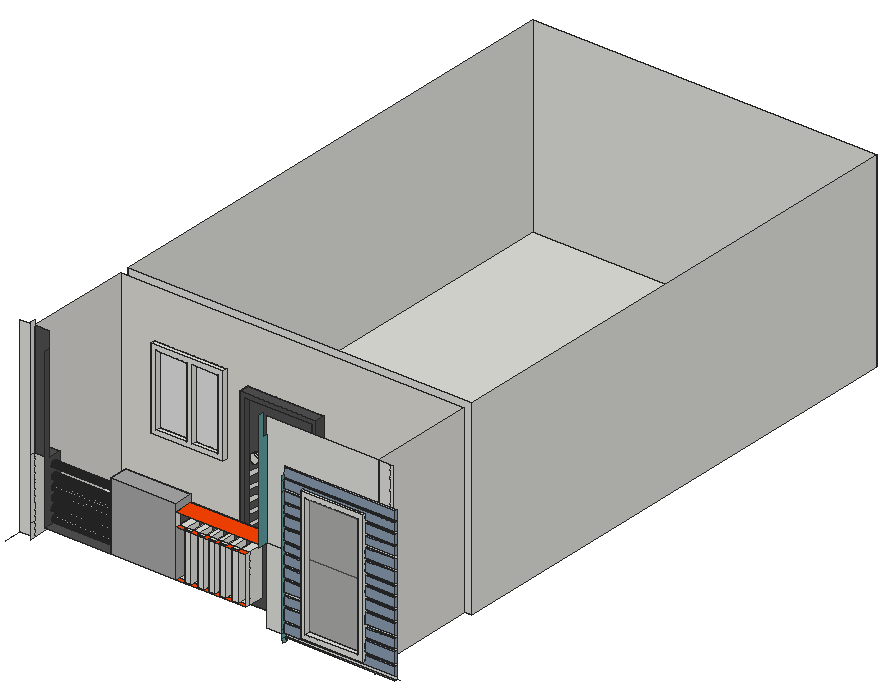
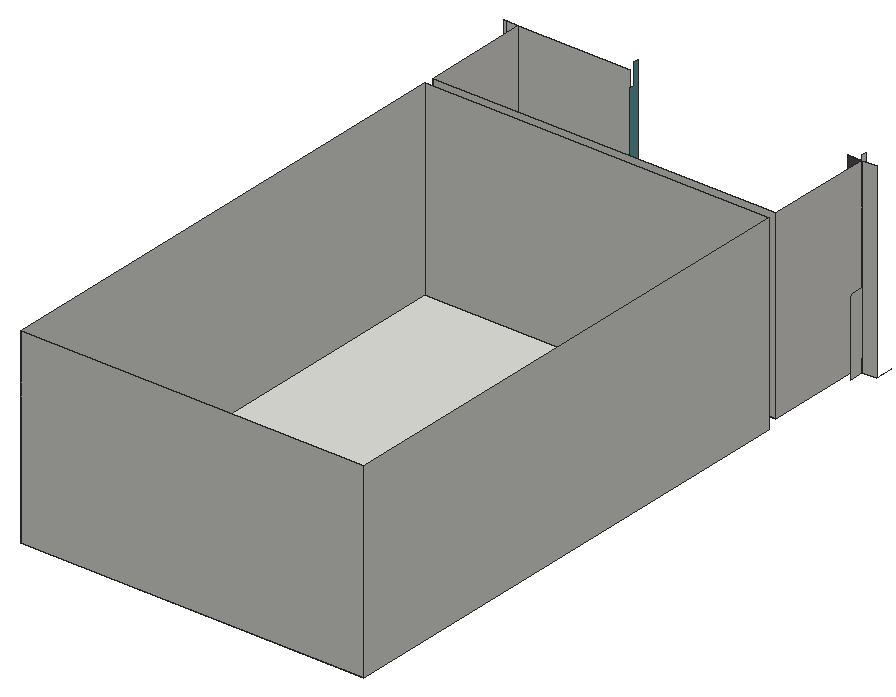
# SketchUp Ruby script. Lengths in inches.
U = 1.inch
M = Sketchup.active_model
def pt(a) = Geom::Point3d.new(a.map { |v| v * U })
def face(e, loops, mat)
  f = e.add_face(loops[0].map { |a| pt(a) })
  loops[1..].each { |l| e.add_face(l.map { |a| pt(a) }).erase! }
  f.material = f.back_material = mat if mat
  f
end
# faces: each face lists its corners as indices into pts; further lists are holes
def faces(e, pts, list, mat = nil) = list.each { |f| face(e, (f[0].is_a?(Array) ? f : [f]).map { |l| l.map { |i| pts[i] } }, mat) }
# xy, xz, yz: faces in a plane at the given z, y or x. An outline is a flat list of corners, or four numbers for a rectangle; further outlines are holes
def ring(l) = l.size == 4 ? [[l[0], l[1]], [l[2], l[1]], [l[2], l[3]], [l[0], l[3]]] : l.each_slice(2).to_a
def flat(e, list, mat, &to3) = list.each { |f| face(e, (f[0].is_a?(Array) ? f : [f]).map { |l| ring(l).map { |u, v| to3.(u, v) } }, mat) }
def xy(e, z, list, mat = nil) = flat(e, list, mat) { |x, y| [x, y, z] }
def xz(e, y, list, mat = nil) = flat(e, list, mat) { |x, z| [x, y, z] }
def yz(e, x, list, mat = nil) = flat(e, list, mat) { |y, z| [x, y, z] }
def lines(e, pts, list) = list.each { |a, b| e.add_line(pt(pts[a]), pt(pts[b])) }
# prism: a flat outline (further loops are holes) pulled along v
def prism(e, loops, v, mat = nil)
  f = face(e, loops, mat); d = Geom::Vector3d.new(v.map { |x| x * U })
  f.pushpull(f.normal.samedirection?(d) ? d.length : -d.length)
end
def box(e, o, s, mat = nil) = prism(e, [[o, [o[0] + s[0], o[1], o[2]], [o[0] + s[0], o[1] + s[1], o[2]], [o[0], o[1] + s[1], o[2]]]], [0, 0, s[2]], mat)
def at(x, y, z, deg = 0) = Geom::Transformation.translation(pt([x, y, z])) * Geom::Transformation.rotation(ORIGIN, Z_AXIS, deg.degrees)
def axes(o, x, y, z) = Geom::Transformation.new([*x, 0, *y, 0, *z, 0, *pt(o).to_a, 1])
def part(name) = M.definitions.add(name)
# library, detail: a bought-in or finely detailed component or shape, given as its bounding box
def library(name, o, s) = part(name).tap { |d| box(d.entities, o, s) }
def detail(e, o, s) = box(e.add_group.entities, o, s)
def put(e, d, t, mat = nil) = e.add_instance(d, t).tap { |i| i.material = mat if mat }
def group(e, t, mat = nil) = e.add_group.tap { |g| g.transformation = t; g.material = mat if mat }.entities
root = M.entities
M.materials.add("[0024_OrangeRed]").color = [255, 69, 0]
M.materials.add("[0081_CadetBlue]").color = [95, 158, 160]
M.materials.add("[0110_LightSlateGray]").color = [139, 158, 178]
M.materials.add("[0132_LightGray]").color = [169, 169, 169]
M.materials.add("[0135_DarkGray]").color = [81, 81, 81]
M.materials.add("[Marble Carrara Gold Floor Tile]").color = [225, 223, 217]
M.materials.add("[Mirror 02]").color = [229, 229, 229]
M.materials.add("[Translucent Glass Gray]").color = [128, 128, 128]
M.materials["[Translucent Glass Gray]"].alpha = 0.5
xy(root,243,[[94.49,73.875,97.49,76.875],[139.49,73.875,142.49,76.875],[94.49,76.875,142.49,79.875],[14,85.875,231.375,405.4375]])
xy(root,244.8,[[175.28,8,245.1875,9]],"[0110_LightSlateGray]")
xy(root,246.6875,[[14,21,231.375,21,231.375,79.875,142.49,79.875,142.49,73.875,139.49,73.875,139.49,76.875,97.49,76.875,97.49,73.875,94.49,73.875,94.49,79.875,14,79.875]])
xy(root,247.25,[[174.92,8,245.1875,9]],"[0110_LightSlateGray]")
xy(root,249.23,[[186.84,6,226.28,8],[186.84,8,226.28,9]])
xy(root,252.23,[[189.84,6,223.28,9]])
xy(root,252.44,[[64.35,9,105.73,12],[110.54,10,114.6,12],[118.66,10,122.72,12],[125.79,10,129.85,12],[132.6,10,136.66,12],
  [140.48,10,144.54,12],[105.73,12,110.54,21],[114.6,12,118.66,21],[122.72,12,125.79,21],[129.85,12,132.6,21],
  [136.66,12,140.48,21],[144.54,12,150.17,21]])
xy(root,252.44,[[105.73,9,150.17,9,150.17,12,144.54,12,144.54,10,140.48,10,140.48,12,136.66,12,136.66,10,132.6,10,132.6,12,129.85,12,129.85,10,125.79,10,125.79,12,122.72,12,122.72,10,118.66,10,118.66,12,114.6,12,114.6,10,110.54,10,110.54,12,105.73,12]],"[0024_OrangeRed]")
xy(root,252.44,[[22.75,9,64.35,21]],"[0135_DarkGray]")
xy(root,252.73,[[174.92,8,186.84,9],[226.28,8,245.1875,9]],"[0110_LightSlateGray]")
xy(root,254.24,[[174.8,8,186.84,9],[226.28,8,245.1875,9]],"[0110_LightSlateGray]")
xy(root,261.28,[[174.8,8,186.84,9],[226.28,8,245.1875,9]],"[0110_LightSlateGray]")
xy(root,262.93,[[174.8,8,186.84,9],[226.28,8,245.1875,9]],"[0110_LightSlateGray]")
xy(root,268.22,[[174.8,8,186.84,9],[226.28,8,245.1875,9]],"[0110_LightSlateGray]")
xy(root,270.4,[[174.8,8,186.84,9],[226.28,8,245.1875,9]],"[0110_LightSlateGray]")
xy(root,276.92,[[174.8,8,186.84,9],[226.28,8,245.1875,9]],"[0110_LightSlateGray]")
xy(root,278.52,[[174.8,8,186.84,9],[226.28,8,245.1875,9]],"[0110_LightSlateGray]")
xy(root,281.07,[[35.8,76.875,80.98,79.875]])
xy(root,282.37,[[110.54,10,114.6,12],[118.66,10,122.72,12],[125.79,10,129.85,12],[132.6,10,136.66,12],[140.48,10,144.54,12],
  [105.73,12,110.54,21],[114.6,12,118.66,21],[122.72,12,125.79,21],[129.85,12,132.6,21],[136.66,12,140.48,21],
  [144.54,12,150.17,21]])
xy(root,282.37,[[105.73,9,105.73,12,110.54,12,110.54,10,114.6,10,114.6,12,118.66,12,118.66,10,122.72,10,122.72,12,125.79,12,125.79,10,129.85,10,129.85,12,132.6,12,132.6,10,136.66,10,136.66,12,140.48,12,140.48,10,144.54,10,144.54,12,150.17,12,150.17,9]],"[0024_OrangeRed]")
xy(root,284.07,[[38.8,76.875,58.39,79.875],[61.35,76.875,77.98,79.875]])
xy(root,284.39,[[174.8,8,186.84,9],[226.28,8,245.1875,9]],"[0110_LightSlateGray]")
xy(root,286,[[174.8,8,186.84,9],[226.28,8,245.1875,9]],"[0110_LightSlateGray]")
xy(root,291,[[105.73,9,105.77,12]])
xy(root,291,[[105.77,9,160.53,9,160.53,12,231.375,12,231.375,21,105.77,21]],"[0024_OrangeRed]")
xy(root,291,[[14,12,22.75,21]],"[0135_DarkGray]")
xy(root,291.74,[[174.8,8,186.84,9],[226.28,8,245.1875,9]],"[0110_LightSlateGray]")
xy(root,293.27,[[226.28,9,245.1875,9.125]])
xy(root,293.27,[[174.8,8,186.84,9],[226.28,8,245.1875,9]],"[0110_LightSlateGray]")
xy(root,295.5625,[[64.35,9,105.77,21]],"[0132_LightGray]")
xy(root,297.89,[[226.28,9,245.1875,9.125]])
xy(root,297.89,[[174.8,8,186.84,9],[226.28,8,245.1875,9]],"[0110_LightSlateGray]")
xy(root,299.48,[[174.8,8,186.84,9],[226.28,8,245.1875,9]],"[0110_LightSlateGray]")
xy(root,306.1,[[174.8,8,186.84,9],[226.28,8,245.1875,9]],"[0110_LightSlateGray]")
xy(root,307.76,[[174.8,8,186.84,9],[226.28,8,245.1875,9]],"[0110_LightSlateGray]")
xy(root,313.43,[[174.8,8,186.84,9],[226.28,8,245.1875,9]],"[0110_LightSlateGray]")
xy(root,315.26,[[174.8,8,186.84,9],[226.28,8,245.1875,9]],"[0110_LightSlateGray]")
xy(root,320.33,[[174.8,8,186.84,9],[226.28,8,245.1875,9]],"[0110_LightSlateGray]")
xy(root,321.68,[[174.8,8,186.84,9],[226.28,8,245.1875,9]],"[0110_LightSlateGray]")
xy(root,324,[[97.49,73.875,139.49,76.875]],"[0135_DarkGray]")
xy(root,327,[[94.49,73.875,142.49,79.875]],"[0135_DarkGray]")
xy(root,327.27,[[174.8,8,186.84,9],[226.28,8,245.1875,9]],"[0110_LightSlateGray]")
xy(root,328.89,[[174.8,8,186.84,9],[226.28,8,245.1875,9]],"[0110_LightSlateGray]")
xy(root,329.07,[[38.8,76.875,58.39,79.875],[61.35,76.875,77.98,79.875]])
xy(root,329.73,[[189.84,6,223.28,9]])
xy(root,332.07,[[35.8,76.875,80.98,79.875]])
xy(root,332.73,[[186.84,6,226.28,8],[186.84,8,226.28,9]])
xy(root,334.1,[[174.8,8,245.1875,9]],"[0110_LightSlateGray]")
xy(root,335.48,[[174.89,8,245.1875,9]],"[0110_LightSlateGray]")
xz(root,6,[[[186.84,249.23,226.28,332.73],[189.84,252.23,223.28,329.73]]])
xz(root,8,[[174.92,247.25,245.1875,247.25,245.1875,252.73,226.28,252.73,226.28,249.23,186.84,249.23,186.84,252.73,174.92,252.73],[174.8,254.24,186.84,261.28],[226.28,254.24,245.1875,261.28],[174.8,262.93,186.84,268.22],[226.28,262.93,245.1875,268.22],
  [174.8,270.4,186.84,276.92],[226.28,270.4,245.1875,276.92],[174.8,278.52,186.84,284.39],[226.28,278.52,245.1875,284.39],[174.8,286,186.84,291.74],
  [226.28,286,245.1875,291.74],[174.8,293.27,186.84,297.89],[226.28,293.27,245.1875,297.89],[174.8,299.48,186.84,306.1],[226.28,299.48,245.1875,306.1],
  [174.8,307.76,186.84,313.43],[226.28,307.76,245.1875,313.43],[174.8,315.26,186.84,320.33],[226.28,315.26,245.1875,320.33],[174.8,321.68,186.84,327.27],
  [226.28,321.68,245.1875,327.27],[174.8,328.89,186.84,328.89,186.84,332.73,226.28,332.73,226.28,328.89,245.1875,328.89,245.1875,334.1,174.8,334.1],[174.89,335.48,245.1875,335.48,245.1875,341.1,176.04,341.1,175.52,339.57,174.98,336.86]],"[0110_LightSlateGray]")
xz(root,9,[[175.28,244.8,245.1875,244.8,245.1875,247.25,174.92,247.25],[174.92,247.25,174.92,252.73,186.84,252.73,186.84,254.24,174.8,254.24,174.8,249.73],[174.92,247.25,174.92,252.73,186.84,252.73,186.84,249.23,226.28,249.23,226.28,252.73,245.1875,252.73,245.1875,247.25],[226.28,252.73,245.1875,254.24],[174.8,254.24,186.84,261.28],
  [226.28,254.24,245.1875,261.28],[174.8,261.28,186.84,262.93],[226.28,261.28,245.1875,262.93],[174.8,262.93,186.84,268.22],[226.28,262.93,245.1875,268.22],
  [174.8,268.22,186.84,270.4],[226.28,268.22,245.1875,270.4],[174.8,270.4,186.84,276.92],[226.28,270.4,245.1875,276.92],[174.8,276.92,186.84,278.52],
  [226.28,276.92,245.1875,278.52],[174.8,278.52,186.84,284.39],[226.28,278.52,245.1875,284.39],[174.8,284.39,186.84,286],[226.28,284.39,245.1875,286],
  [174.8,286,186.84,291.74],[226.28,286,245.1875,291.74],[174.8,291.74,186.84,293.27],[226.28,291.74,245.1875,293.27],[174.8,293.27,186.84,297.89],
  [174.8,297.89,186.84,299.48],[226.28,297.89,245.1875,299.48],[174.8,299.48,186.84,306.1],[226.28,299.48,245.1875,306.1],[174.8,306.1,186.84,307.76],
  [226.28,306.1,245.1875,307.76],[174.8,307.76,186.84,313.43],[226.28,307.76,245.1875,313.43],[174.8,313.43,186.84,315.26],[226.28,313.43,245.1875,315.26],
  [174.8,315.26,186.84,320.33],[226.28,315.26,245.1875,320.33],[174.8,320.33,186.84,321.68],[226.28,320.33,245.1875,321.68],[174.8,321.68,186.84,327.27],
  [226.28,321.68,245.1875,327.27],[174.8,327.27,186.84,328.89],[226.28,327.27,245.1875,328.89],[174.8,328.89,174.8,334.1,245.1875,334.1,245.1875,328.89,226.28,328.89,226.28,332.73,186.84,332.73,186.84,328.89],[174.8,334.1,245.1875,334.1,245.1875,335.48,174.89,335.48],
  [174.89,335.48,174.98,336.86,175.52,339.57,176.04,341.1,174.89,341.1],[174.89,335.48,174.98,336.86,175.52,339.57,176.04,341.1,245.1875,341.1,245.1875,335.48]])
xz(root,9,[[64.35,252.44,105.73,252.44,105.73,291,105.77,291,105.77,295.5625,64.35,295.5625]],"[0132_LightGray]")
xz(root,9,[[189.84,252.23,223.28,329.73]],"[Translucent Glass Gray]")
xz(root,9.125,[[226.28,293.27,245.1875,297.89]])
xz(root,10,[[110.54,252.44,114.6,282.37],[118.66,252.44,122.72,282.37],[125.79,252.44,129.85,282.37],[132.6,252.44,136.66,282.37],[140.48,252.44,144.54,282.37]])
xz(root,12,[[5,243,14,363],[160.53,243,231.375,291],[231.375,243,238.75,363],[238.75,243,240.375,363],[160.53,291,231.375,363]])
xz(root,12,[[14,291,22.75,363]],"[0135_DarkGray]")
xz(root,21,[[[14,246.6875,14,291,22.75,291,22.75,252.44,64.35,252.44,64.35,295.5625,105.77,295.5625,105.77,291,231.375,291,231.375,246.6875],[144.54,252.44,150.17,282.37],[105.73,252.44,110.54,282.37],[114.6,252.44,118.66,282.37],[136.66,252.44,140.48,282.37],[122.72,252.44,125.79,282.37],[129.85,252.44,132.6,282.37]]],"[0135_DarkGray]")
xz(root,73.875,[[94.49,243,97.49,246.6875],[139.49,243,142.49,246.6875],[103.24,288.58,103.98,288.67,104.68,288.96,105.27,289.42,105.73,290.01,106.02,290.71,106.12,291.45,106.02,292.19,105.73,292.89,105.27,293.48,104.68,293.94,103.98,294.23,103.24,294.33,102.5,294.23,101.8,293.94,101.21,293.48,100.75,292.89,100.46,292.19,100.37,291.45,100.46,290.71,100.75,290.01,101.21,289.42,101.8,288.96,102.5,288.67]])
xz(root,73.875,[[94.49,246.6875,97.49,246.6875,97.49,324,139.49,324,139.49,246.6875,142.49,246.6875,142.49,327,94.49,327]],"[0135_DarkGray]")
xz(root,76.875,[[97.49,242.7,97.88,243,97.49,243],[97.49,243,97.88,243,97.88,245.43,97.49,245.13],[97.88,243,103.74,243,103.74,246.6875,102.62,246.6875],[97.88,243,97.88,245.43,99.52,246.6875,102.62,246.6875],[103.74,243,106.79,245.35,106.79,243],
  [103.74,243,106.79,245.35,106.79,246.6875,103.74,246.6875],[106.79,243,106.79,245.35,108.52,246.6875,111.53,246.6875],[106.79,243,139.49,243,139.49,246.6875,111.53,246.6875],[97.49,245.13,97.49,246.6875,97.88,246.6875,97.88,245.43],[106.79,245.35,106.79,246.6875,108.52,246.6875],
  [97.88,245.43,97.88,246.6875,99.52,246.6875],[99.52,246.6875,102.62,246.6875,139.49,275.41,139.49,277.48],[108.52,246.6875,111.53,246.6875,139.49,268.47,139.49,270.54],[97.49,249.63,139.49,282.34,139.49,284.41,97.49,252.07],[97.49,256.57,139.49,289.28,139.49,291.35,97.49,259],
  [97.49,263.51,139.49,296.22,139.49,298.29,97.49,265.94],[97.49,270.45,139.49,303.16,139.49,305.23,97.49,272.88],[97.49,278.22,139.49,310.93,139.49,313,97.49,280.65],[[35.8,281.07,80.98,332.07],[38.8,284.07,58.39,329.07],[61.35,284.07,77.98,329.07]]])
xz(root,76.875,[[97.49,246.6875,99.52,246.6875,139.49,277.48,139.49,282.34,97.49,249.63],[102.62,246.6875,108.52,246.6875,139.49,270.54,139.49,275.41],[111.53,246.6875,139.49,246.6875,139.49,268.47],[97.49,252.07,139.49,284.41,139.49,289.28,97.49,256.57],[97.49,259,139.49,291.35,139.49,296.22,97.49,263.51],
  [97.49,265.94,139.49,298.29,139.49,303.16,97.49,270.45],[97.49,272.88,139.49,305.23,139.49,310.93,97.49,278.22],[[97.49,280.65,139.49,313,139.49,324,97.49,324],[103.24,288.58,102.5,288.67,101.8,288.96,101.21,289.42,100.75,290.01,100.46,290.71,100.37,291.45,100.46,292.19,100.75,292.89,101.21,293.48,101.8,293.94,102.5,294.23,103.24,294.33,103.98,294.23,104.68,293.94,105.27,293.48,105.73,292.89,106.02,292.19,106.12,291.45,106.02,290.71,105.73,290.01,105.27,289.42,104.68,288.96,103.98,288.67]]],"[0135_DarkGray]")
xz(root,79.875,[[94.49,243,142.49,327],[[35.8,281.07,80.98,332.07],[38.8,284.07,58.39,329.07],[61.35,284.07,77.98,329.07]]])
xz(root,79.875,[[[14,246.6875,94.49,246.6875,94.49,327,142.49,327,142.49,246.6875,231.375,246.6875,231.375,363,14,363],[35.8,281.07,80.98,332.07]]],"[Marble Carrara Gold Floor Tile]")
xz(root,79.875,[[38.8,284.07,58.39,329.07],[61.35,284.07,77.98,329.07]],"[Mirror 02]")
xz(root,85.875,[[14,243,231.375,363]])
xz(root,405.4375,[[14,243,231.375,363]])
yz(root,14,[[9,243,12,252.44],[12,243,21,291],[85.875,243,405.4375,363],[9,252.44,12,291],[9,291,12,366]])
yz(root,14,[[21,246.6875,79.875,246.6875,79.875,363,12,363,12,291,21,291]],"[Marble Carrara Gold Floor Tile]")
yz(root,22.75,[[[9,252.44,21,252.44,21,291,12,291,12,352.5,9,352.5],[15.78,277.4,15.27,277.47,14.78,277.67,14.37,277.98,14.05,278.4,13.85,278.88,13.78,279.4,13.85,279.92,14.05,280.4,14.37,280.8125,14.78,281.13,15.27,281.33,15.78,281.4,16.3,281.33,16.78,281.13,17.2,280.8125,17.52,280.4,17.72,279.92,17.78,279.4,17.72,278.88,17.52,278.4,17.2,277.98,16.78,277.67,16.3,277.47],[15.78,271.4,15.27,271.47,14.78,271.67,14.37,271.98,14.05,272.4,13.85,272.88,13.78,273.4,13.85,273.92,14.05,274.4,14.37,274.8125,14.78,275.13,15.27,275.33,15.78,275.4,16.3,275.33,16.78,275.13,17.2,274.8125,17.52,274.4,17.72,273.92,17.78,273.4,17.72,272.88,17.52,272.4,17.2,271.98,16.78,271.67,16.3,271.47],[15.78,265.4,15.27,265.47,14.78,265.67,14.37,265.98,14.05,266.4,13.85,266.88,13.78,267.4,13.85,267.92,14.05,268.4,14.37,268.8125,14.78,269.13,15.27,269.33,15.78,269.4,16.3,269.33,16.78,269.13,17.2,268.8125,17.52,268.4,17.72,267.92,17.78,267.4,17.72,266.88,17.52,266.4,17.2,265.98,16.78,265.67,16.3,265.47],[15.78,259.4,15.27,259.47,14.78,259.67,14.37,259.98,14.05,260.4,13.85,260.88,13.78,261.4,13.85,261.92,14.05,262.4,14.37,262.8125,14.78,263.13,15.27,263.33,15.78,263.4,16.3,263.33,16.78,263.13,17.2,262.8125,17.52,262.4,17.72,261.92,17.78,261.4,17.72,260.88,17.52,260.4,17.2,259.98,16.78,259.67,16.3,259.47],[15.78,253.4,15.27,253.47,14.78,253.67,14.37,253.98,14.05,254.4,13.85,254.88,13.78,255.4,13.85,255.92,14.05,256.4,14.37,256.8125,14.78,257.13,15.27,257.33,15.78,257.4,16.3,257.33,16.78,257.13,17.2,256.8125,17.52,256.4,17.72,255.92,17.78,255.4,17.72,254.88,17.52,254.4,17.2,253.98,16.78,253.67,16.3,253.47],[15.78,284.27,15.27,284.34,14.78,284.54,14.37,284.86,14.05,285.27,13.85,285.76,13.78,286.27,13.85,286.79,14.05,287.27,14.37,287.6875,14.78,288.01,15.27,288.21,15.78,288.27,16.3,288.21,16.78,288.01,17.2,287.6875,17.52,287.27,17.72,286.79,17.78,286.27,17.72,285.76,17.52,285.27,17.2,284.86,16.78,284.54,16.3,284.34]]],"[0135_DarkGray]")
yz(root,35.8,[[76.875,281.07,79.875,332.07]])
yz(root,38.8,[[76.875,284.07,79.875,329.07]])
yz(root,58.39,[[76.875,284.07,79.875,329.07]])
yz(root,61.35,[[76.875,284.07,79.875,329.07]])
yz(root,64.35,[[9,252.44,21,295.5625]],"[0132_LightGray]")
yz(root,66,[[15.78,277.4,16.3,277.47,16.78,277.67,17.2,277.98,17.52,278.4,17.72,278.88,17.78,279.4,17.72,279.92,17.52,280.4,17.2,280.8125,16.78,281.13,16.3,281.33,15.78,281.4,15.27,281.33,14.78,281.13,14.37,280.8125,14.05,280.4,13.85,279.92,13.78,279.4,13.85,278.88,14.05,278.4,14.37,277.98,14.78,277.67,15.27,277.47]])
yz(root,66.875,[[15.78,253.4,16.3,253.47,16.78,253.67,17.2,253.98,17.52,254.4,17.72,254.88,17.78,255.4,17.72,255.92,17.52,256.4,17.2,256.8125,16.78,257.13,16.3,257.33,15.78,257.4,15.27,257.33,14.78,257.13,14.37,256.8125,14.05,256.4,13.85,255.92,13.78,255.4,13.85,254.88,14.05,254.4,14.37,253.98,14.78,253.67,15.27,253.47]])
yz(root,67.5625,[[15.78,259.4,16.3,259.47,16.78,259.67,17.2,259.98,17.52,260.4,17.72,260.88,17.78,261.4,17.72,261.92,17.52,262.4,17.2,262.8125,16.78,263.13,16.3,263.33,15.78,263.4,15.27,263.33,14.78,263.13,14.37,262.8125,14.05,262.4,13.85,261.92,13.78,261.4,13.85,260.88,14.05,260.4,14.37,259.98,14.78,259.67,15.27,259.47]])
yz(root,67.8125,[[15.78,265.4,16.3,265.47,16.78,265.67,17.2,265.98,17.52,266.4,17.72,266.88,17.78,267.4,17.72,267.92,17.52,268.4,17.2,268.8125,16.78,269.13,16.3,269.33,15.78,269.4,15.27,269.33,14.78,269.13,14.37,268.8125,14.05,268.4,13.85,267.92,13.78,267.4,13.85,266.88,14.05,266.4,14.37,265.98,14.78,265.67,15.27,265.47],[15.78,271.4,16.3,271.47,16.78,271.67,17.2,271.98,17.52,272.4,17.72,272.88,17.78,273.4,17.72,273.92,17.52,274.4,17.2,274.8125,16.78,275.13,16.3,275.33,15.78,275.4,15.27,275.33,14.78,275.13,14.37,274.8125,14.05,274.4,13.85,273.92,13.78,273.4,13.85,272.88,14.05,272.4,14.37,271.98,14.78,271.67,15.27,271.47]])
yz(root,68.0625,[[15.78,284.27,16.3,284.34,16.78,284.54,17.2,284.86,17.52,285.27,17.72,285.76,17.78,286.27,17.72,286.79,17.52,287.27,17.2,287.6875,16.78,288.01,16.3,288.21,15.78,288.27,15.27,288.21,14.78,288.01,14.37,287.6875,14.05,287.27,13.85,286.79,13.78,286.27,13.85,285.76,14.05,285.27,14.37,284.86,14.78,284.54,15.27,284.34]])
yz(root,77.98,[[76.875,284.07,79.875,329.07]])
yz(root,80.98,[[76.875,281.07,79.875,332.07]])
yz(root,94.49,[[73.875,243,76.875,246.6875],[76.875,243,79.875,246.6875]])
yz(root,94.49,[[73.875,246.6875,79.875,327]],"[0135_DarkGray]")
yz(root,97.49,[[73.875,243,76.875,246.6875]])
yz(root,97.49,[[73.875,246.6875,76.875,324]],"[0135_DarkGray]")
yz(root,105.73,[[9,282.37,12,291]])
yz(root,105.73,[[9,252.44,21,282.37]],"[0132_LightGray]")
yz(root,105.77,[[9,291,21,295.5625]],"[0132_LightGray]")
yz(root,110.54,[[10,252.44,21,282.37]])
yz(root,114.6,[[10,252.44,21,282.37]])
yz(root,118.66,[[10,252.44,21,282.37]])
yz(root,122.72,[[10,252.44,21,282.37]])
yz(root,125.79,[[10,252.44,21,282.37]])
yz(root,129.85,[[10,252.44,21,282.37]])
yz(root,132.6,[[10,252.44,21,282.37]])
yz(root,136.66,[[10,252.44,21,282.37]])
yz(root,139.49,[[73.875,243,76.875,246.6875]])
yz(root,139.49,[[73.875,246.6875,76.875,324]],"[0135_DarkGray]")
yz(root,140.48,[[10,252.44,21,282.37]])
yz(root,142.49,[[73.875,243,76.875,246.6875],[76.875,243,79.875,246.6875]])
yz(root,142.49,[[73.875,246.6875,79.875,327]],"[0135_DarkGray]")
yz(root,144.54,[[10,252.44,21,282.37]])
yz(root,150.17,[[9,252.44,12,282.37],[12,252.44,21,282.37]])
yz(root,160.53,[[6,291,6,366,9,366,9,352.5,12,352.5,12,291]],"[0081_CadetBlue]")
yz(root,174.8,[[8,254.24,9,261.28],[8,262.93,9,268.22],[8,270.4,9,276.92],[8,278.52,9,284.39],[8,286,9,291.74],
  [8,293.27,9,297.89],[8,299.48,9,306.1],[8,307.76,9,313.43],[8,315.26,9,320.33],[8,321.68,9,327.27],
  [8,328.89,9,334.1]])
yz(root,174.8,[[6,249.73,9,249.73,9,254.24,8,254.24,8,261.28,9,261.28,9,262.93,8,262.93,8,268.22,9,268.22,9,270.4,8,270.4,8,276.92,9,276.92,9,278.52,8,278.52,8,284.39,9,284.39,9,286,8,286,8,291.74,9,291.74,9,293.27,8,293.27,8,297.89,9,297.89,9,299.48,8,299.48,8,306.1,9,306.1,9,307.76,8,307.76,8,313.43,9,313.43,9,315.26,8,315.26,8,320.33,9,320.33,9,321.68,8,321.68,8,327.27,6,327.27],[6,327.27,9,327.27,9,328.89,8,328.89,8,334.1,6,334.1]],"[0081_CadetBlue]")
yz(root,174.92,[[8,247.25,9,252.73]])
yz(root,186.84,[[6,249.23,6,332.73,8,332.73,8,328.89,9,328.89,9,327.27,8,327.27,8,321.68,9,321.68,9,320.33,8,320.33,8,315.26,9,315.26,9,313.43,8,313.43,8,307.76,9,307.76,9,306.1,8,306.1,8,299.48,9,299.48,9,297.89,8,297.89,8,293.27,9,293.27,9,291.74,8,291.74,8,286,9,286,9,284.39,8,284.39,8,278.52,9,278.52,9,276.92,8,276.92,8,270.4,9,270.4,9,268.22,8,268.22,8,262.93,9,262.93,9,261.28,8,261.28,8,254.24,9,254.24,9,252.73,8,252.73,8,249.23],[8,249.23,9,252.73],[8,254.24,9,261.28],[8,262.93,9,268.22],[8,270.4,9,276.92],
  [8,278.52,9,284.39],[8,286,9,291.74],[8,293.27,9,297.89],[8,299.48,9,306.1],[8,307.76,9,313.43],
  [8,315.26,9,320.33],[8,321.68,9,327.27],[8,328.89,9,332.73]])
yz(root,189.84,[[6,252.23,9,329.73]])
yz(root,223.28,[[6,252.23,9,329.73]])
yz(root,226.28,[[6,249.23,8,249.23,8,252.73,9,252.73,9,254.24,8,254.24,8,261.28,9,261.28,9,262.93,8,262.93,8,268.22,9,268.22,9,270.4,8,270.4,8,276.92,9,276.92,9,278.52,8,278.52,8,284.39,9,284.39,9,286,8,286,8,291.74,9,291.74,9,293.27,8,293.27,8,297.89,9,297.89,9,299.48,8,299.48,8,306.1,9,306.1,9,307.76,8,307.76,8,313.43,9,313.43,9,315.26,8,315.26,8,320.33,9,320.33,9,321.68,8,321.68,8,327.27,9,327.27,9,328.89,8,328.89,8,332.73,6,332.73],[8,249.23,9,252.73],[8,254.24,9,261.28],[8,262.93,9,268.22],[8,270.4,9,276.92],
  [8,278.52,9,284.39],[8,286,9,291.74],[8,293.27,9,297.89],[9,293.27,9.125,297.89],[8,299.48,9,306.1],
  [8,307.76,9,313.43],[8,315.26,9,320.33],[8,321.68,9,327.27],[8,328.89,9,332.73]])
yz(root,231.375,[[12,243,21,291],[85.875,243,405.4375,363]])
yz(root,231.375,[[21,246.6875,21,291,12,291,12,363,79.875,363,79.875,246.6875]],"[Marble Carrara Gold Floor Tile]")
yz(root,245.1875,[[8,247.25,9,252.73],[8,254.24,9,261.28],[8,262.93,9,268.22],[8,270.4,9,276.92],[8,278.52,9,284.39],
  [8,286,9,291.74],[8,293.27,9.125,297.89],[8,299.48,9,306.1],[8,307.76,9,313.43],[8,315.26,9,320.33],
  [8,321.68,9,327.27],[8,328.89,9,334.1],[8,335.48,9,341.1]],"[0110_LightSlateGray]")
p = [[175.87,6,242.4],[175.87,8,242.4],[175.28,8,244.8],[175.28,6,244.8],[175.87,9,242.4],[175.28,9,244.8],
  [174.92,9,247.25],[174.92,8,247.25],[174.92,6,247.25],[174.8,9,249.73],[174.8,6,249.73],[22.75,15.27,253.47],
  [22.75,15.78,253.4],[66.875,15.78,253.4],[66.875,15.27,253.47],[22.75,16.3,253.47],[66.875,16.3,253.47],[22.75,14.78,253.67],
  [66.875,14.78,253.67],[22.75,16.78,253.67],[66.875,16.78,253.67],[22.75,14.37,253.98],[66.875,14.37,253.98],[22.75,17.2,253.98],
  [66.875,17.2,253.98],[22.75,14.05,254.4],[66.875,14.05,254.4],[22.75,17.52,254.4],[66.875,17.52,254.4],[22.75,13.85,254.88],
  [66.875,13.85,254.88],[22.75,17.72,254.88],[66.875,17.72,254.88],[22.75,13.78,255.4],[66.875,13.78,255.4],[22.75,17.78,255.4],
  [66.875,17.78,255.4],[22.75,13.85,255.92],[66.875,13.85,255.92],[22.75,17.72,255.92],[66.875,17.72,255.92],[22.75,14.05,256.4],
  [66.875,14.05,256.4],[22.75,17.52,256.4],[66.875,17.52,256.4],[22.75,14.37,256.8125],[66.875,14.37,256.8125],[22.75,17.2,256.8125],
  [66.875,17.2,256.8125],[22.75,14.78,257.13],[66.875,14.78,257.13],[22.75,16.78,257.13],[66.875,16.78,257.13],[22.75,15.27,257.33],
  [66.875,15.27,257.33],[22.75,16.3,257.33],[66.875,16.3,257.33],[22.75,15.78,257.4],[66.875,15.78,257.4],[22.75,15.27,259.47],
  [22.75,15.78,259.4],[67.5625,15.78,259.4],[67.5625,15.27,259.47],[22.75,16.3,259.47],[67.5625,16.3,259.47],[22.75,14.78,259.67],
  [67.5625,14.78,259.67],[22.75,16.78,259.67],[67.5625,16.78,259.67],[22.75,14.37,259.98],[67.5625,14.37,259.98],[22.75,17.2,259.98],
  [67.5625,17.2,259.98],[22.75,14.05,260.4],[67.5625,14.05,260.4],[22.75,17.52,260.4],[67.5625,17.52,260.4],[22.75,13.85,260.88],
  [67.5625,13.85,260.88],[22.75,17.72,260.88],[67.5625,17.72,260.88],[22.75,13.78,261.4],[67.5625,13.78,261.4],[22.75,17.78,261.4],
  [67.5625,17.78,261.4],[22.75,13.85,261.92],[67.5625,13.85,261.92],[22.75,17.72,261.92],[67.5625,17.72,261.92],[22.75,14.05,262.4],
  [67.5625,14.05,262.4],[22.75,17.52,262.4],[67.5625,17.52,262.4],[22.75,14.37,262.8125],[67.5625,14.37,262.8125],[22.75,17.2,262.8125],
  [67.5625,17.2,262.8125],[22.75,14.78,263.13],[67.5625,14.78,263.13],[22.75,16.78,263.13],[67.5625,16.78,263.13],[22.75,15.27,263.33],
  [67.5625,15.27,263.33],[22.75,16.3,263.33],[67.5625,16.3,263.33],[22.75,15.78,263.4],[67.5625,15.78,263.4],[22.75,15.27,265.47],
  [22.75,15.78,265.4],[67.8125,15.78,265.4],[67.8125,15.27,265.47],[22.75,16.3,265.47],[67.8125,16.3,265.47],[22.75,14.78,265.67],
  [67.8125,14.78,265.67],[22.75,16.78,265.67],[67.8125,16.78,265.67],[22.75,14.37,265.98],[67.8125,14.37,265.98],[22.75,17.2,265.98],
  [67.8125,17.2,265.98],[22.75,14.05,266.4],[67.8125,14.05,266.4],[22.75,17.52,266.4],[67.8125,17.52,266.4],[22.75,13.85,266.88],
  [67.8125,13.85,266.88],[22.75,17.72,266.88],[67.8125,17.72,266.88],[22.75,13.78,267.4],[67.8125,13.78,267.4],[22.75,17.78,267.4],
  [67.8125,17.78,267.4],[22.75,13.85,267.92],[67.8125,13.85,267.92],[22.75,17.72,267.92],[67.8125,17.72,267.92],[22.75,14.05,268.4],
  [67.8125,14.05,268.4],[22.75,17.52,268.4],[67.8125,17.52,268.4],[22.75,14.37,268.8125],[67.8125,14.37,268.8125],[22.75,17.2,268.8125],
  [67.8125,17.2,268.8125],[22.75,14.78,269.13],[67.8125,14.78,269.13],[22.75,16.78,269.13],[67.8125,16.78,269.13],[22.75,15.27,269.33],
  [67.8125,15.27,269.33],[22.75,16.3,269.33],[67.8125,16.3,269.33],[22.75,15.78,269.4],[67.8125,15.78,269.4],[22.75,15.27,271.47],
  [22.75,15.78,271.4],[67.8125,15.78,271.4],[67.8125,15.27,271.47],[22.75,16.3,271.47],[67.8125,16.3,271.47],[22.75,14.78,271.67],
  [67.8125,14.78,271.67],[22.75,16.78,271.67],[67.8125,16.78,271.67],[22.75,14.37,271.98],[67.8125,14.37,271.98],[22.75,17.2,271.98],
  [67.8125,17.2,271.98],[22.75,14.05,272.4],[67.8125,14.05,272.4],[22.75,17.52,272.4],[67.8125,17.52,272.4],[22.75,13.85,272.88],
  [67.8125,13.85,272.88],[22.75,17.72,272.88],[67.8125,17.72,272.88],[22.75,13.78,273.4],[67.8125,13.78,273.4],[22.75,17.78,273.4],
  [67.8125,17.78,273.4],[22.75,13.85,273.92],[67.8125,13.85,273.92],[22.75,17.72,273.92],[67.8125,17.72,273.92],[22.75,14.05,274.4],
  [67.8125,14.05,274.4],[22.75,17.52,274.4],[67.8125,17.52,274.4],[22.75,14.37,274.8125],[67.8125,14.37,274.8125],[22.75,17.2,274.8125],
  [67.8125,17.2,274.8125],[22.75,14.78,275.13],[67.8125,14.78,275.13],[22.75,16.78,275.13],[67.8125,16.78,275.13],[22.75,15.27,275.33],
  [67.8125,15.27,275.33],[22.75,16.3,275.33],[67.8125,16.3,275.33],[22.75,15.78,275.4],[67.8125,15.78,275.4],[22.75,15.27,277.47],
  [22.75,15.78,277.4],[66,15.78,277.4],[66,15.27,277.47],[22.75,16.3,277.47],[66,16.3,277.47],[22.75,14.78,277.67],
  [66,14.78,277.67],[22.75,16.78,277.67],[66,16.78,277.67],[22.75,14.37,277.98],[66,14.37,277.98],[22.75,17.2,277.98],
  [66,17.2,277.98],[22.75,14.05,278.4],[66,14.05,278.4],[22.75,17.52,278.4],[66,17.52,278.4],[22.75,13.85,278.88],
  [66,13.85,278.88],[22.75,17.72,278.88],[66,17.72,278.88],[22.75,13.78,279.4],[66,13.78,279.4],[22.75,17.78,279.4],
  [66,17.78,279.4],[22.75,13.85,279.92],[66,13.85,279.92],[22.75,17.72,279.92],[66,17.72,279.92],[22.75,14.05,280.4],
  [66,14.05,280.4],[22.75,17.52,280.4],[66,17.52,280.4],[22.75,14.37,280.8125],[66,14.37,280.8125],[22.75,17.2,280.8125],
  [66,17.2,280.8125],[22.75,14.78,281.13],[66,14.78,281.13],[22.75,16.78,281.13],[66,16.78,281.13],[22.75,15.27,281.33],
  [66,15.27,281.33],[22.75,16.3,281.33],[66,16.3,281.33],[22.75,15.78,281.4],[66,15.78,281.4],[22.75,14.78,284.54],
  [22.75,15.27,284.34],[68.0625,15.27,284.34],[68.0625,14.78,284.54],[22.75,15.78,284.27],[68.0625,15.78,284.27],[22.75,16.3,284.34],
  [68.0625,16.3,284.34],[22.75,16.78,284.54],[68.0625,16.78,284.54],[22.75,14.37,284.86],[68.0625,14.37,284.86],[22.75,17.2,284.86],
  [68.0625,17.2,284.86],[22.75,14.05,285.27],[68.0625,14.05,285.27],[22.75,17.52,285.27],[68.0625,17.52,285.27],[22.75,13.85,285.76],
  [68.0625,13.85,285.76],[22.75,17.72,285.76],[68.0625,17.72,285.76],[22.75,13.78,286.27],[68.0625,13.78,286.27],[22.75,17.78,286.27],
  [68.0625,17.78,286.27],[22.75,13.85,286.79],[68.0625,13.85,286.79],[22.75,17.72,286.79],[68.0625,17.72,286.79],[22.75,14.05,287.27],
  [68.0625,14.05,287.27],[22.75,17.52,287.27],[68.0625,17.52,287.27],[22.75,14.37,287.6875],[68.0625,14.37,287.6875],[22.75,17.2,287.6875],
  [68.0625,17.2,287.6875],[22.75,14.78,288.01],[68.0625,14.78,288.01],[22.75,16.78,288.01],[68.0625,16.78,288.01],[22.75,15.27,288.21],
  [68.0625,15.27,288.21],[22.75,16.3,288.21],[68.0625,16.3,288.21],[22.75,15.78,288.27],[68.0625,15.78,288.27],[102.5,76.875,288.67],
  [103.24,76.875,288.58],[103.24,73.875,288.58],[102.5,73.875,288.67],[103.98,76.875,288.67],[103.98,73.875,288.67],[101.8,76.875,288.96],
  [101.8,73.875,288.96],[104.68,76.875,288.96],[104.68,73.875,288.96],[101.21,76.875,289.42],[101.21,73.875,289.42],[105.27,76.875,289.42],
  [105.27,73.875,289.42],[100.75,76.875,290.01],[100.75,73.875,290.01],[105.73,76.875,290.01],[105.73,73.875,290.01],[100.46,76.875,290.71],
  [100.46,73.875,290.71],[106.02,76.875,290.71],[106.02,73.875,290.71],[100.37,76.875,291.45],[100.37,73.875,291.45],[106.12,76.875,291.45],
  [106.12,73.875,291.45],[100.46,76.875,292.19],[100.46,73.875,292.19],[106.02,76.875,292.19],[106.02,73.875,292.19],[100.75,76.875,292.89],
  [100.75,73.875,292.89],[105.73,76.875,292.89],[105.73,73.875,292.89],[101.21,76.875,293.48],[101.21,73.875,293.48],[105.27,76.875,293.48],
  [105.27,73.875,293.48],[101.8,76.875,293.94],[101.8,73.875,293.94],[104.68,76.875,293.94],[104.68,73.875,293.94],[102.5,76.875,294.23],
  [102.5,73.875,294.23],[103.98,76.875,294.23],[103.98,73.875,294.23],[103.24,76.875,294.33],[103.24,73.875,294.33],[174.8,9,334.1],
  [174.89,9,335.48],[174.89,8,335.48],[174.98,8,336.86],[174.98,6,336.86],[174.8,6,334.1],[174.8,8,334.1],
  [174.98,9,336.86],[231.375,12,243],[231.375,9,243],[241.9375,12,243],[245.1875,12,243],[5,12,243],
  [5,0,243]]
faces(root,p,[[0,1,2,3],[5,6,7,8,3,2],[6,9,10,8,7],[347,348,349,350,351,352,353]],"[0081_CadetBlue]")
faces(root,p,[[4,5,2,1],[299,300,301,302],[300,303,304,301],[305,299,302,306],[303,307,308,304],[309,305,306,310],[307,311,312,308],[313,309,310,314],
  [311,315,316,312],[317,313,314,318],[315,319,320,316],[321,317,318,322],[319,323,324,320],[325,321,322,326],[323,327,328,324],[329,325,326,330],
  [327,331,332,328],[333,329,330,334],[331,335,336,332],[337,333,334,338],[335,339,340,336],[341,337,338,342],[339,343,344,340],[345,341,342,346],
  [343,345,346,344],[348,354,350,349]])
faces(root,p,[[11,12,13,14],[12,15,16,13],[17,11,14,18],[15,19,20,16],[21,17,18,22],[19,23,24,20],[25,21,22,26],[23,27,28,24],
  [29,25,26,30],[27,31,32,28],[33,29,30,34],[31,35,36,32],[37,33,34,38],[35,39,40,36],[41,37,38,42],[39,43,44,40],
  [45,41,42,46],[43,47,48,44],[49,45,46,50],[47,51,52,48],[53,49,50,54],[51,55,56,52],[57,53,54,58],[55,57,58,56],
  [59,60,61,62],[60,63,64,61],[65,59,62,66],[63,67,68,64],[69,65,66,70],[67,71,72,68],[73,69,70,74],[71,75,76,72],
  [77,73,74,78],[75,79,80,76],[81,77,78,82],[79,83,84,80],[85,81,82,86],[83,87,88,84],[89,85,86,90],[87,91,92,88],
  [93,89,90,94],[91,95,96,92],[97,93,94,98],[95,99,100,96],[101,97,98,102],[99,103,104,100],[105,101,102,106],[103,105,106,104],
  [107,108,109,110],[108,111,112,109],[113,107,110,114],[111,115,116,112],[117,113,114,118],[115,119,120,116],[121,117,118,122],[119,123,124,120],
  [125,121,122,126],[123,127,128,124],[129,125,126,130],[127,131,132,128],[133,129,130,134],[131,135,136,132],[137,133,134,138],[135,139,140,136],
  [141,137,138,142],[139,143,144,140],[145,141,142,146],[143,147,148,144],[149,145,146,150],[147,151,152,148],[153,149,150,154],[151,153,154,152],
  [155,156,157,158],[156,159,160,157],[161,155,158,162],[159,163,164,160],[165,161,162,166],[163,167,168,164],[169,165,166,170],[167,171,172,168],
  [173,169,170,174],[171,175,176,172],[177,173,174,178],[175,179,180,176],[181,177,178,182],[179,183,184,180],[185,181,182,186],[183,187,188,184],
  [189,185,186,190],[187,191,192,188],[193,189,190,194],[191,195,196,192],[197,193,194,198],[195,199,200,196],[201,197,198,202],[199,201,202,200],
  [203,204,205,206],[204,207,208,205],[209,203,206,210],[207,211,212,208],[213,209,210,214],[211,215,216,212],[217,213,214,218],[215,219,220,216],
  [221,217,218,222],[219,223,224,220],[225,221,222,226],[223,227,228,224],[229,225,226,230],[227,231,232,228],[233,229,230,234],[231,235,236,232],
  [237,233,234,238],[235,239,240,236],[241,237,238,242],[239,243,244,240],[245,241,242,246],[243,247,248,244],[249,245,246,250],[247,249,250,248],
  [251,252,253,254],[252,255,256,253],[255,257,258,256],[257,259,260,258],[261,251,254,262],[259,263,264,260],[265,261,262,266],[263,267,268,264],
  [269,265,266,270],[267,271,272,268],[273,269,270,274],[271,275,276,272],[277,273,274,278],[275,279,280,276],[281,277,278,282],[279,283,284,280],
  [285,281,282,286],[283,287,288,284],[289,285,286,290],[287,291,292,288],[293,289,290,294],[291,295,296,292],[297,293,294,298],[295,297,298,296]],"[0132_LightGray]")
lines(root,p,[[355,356],[357,358],[359,360]])
